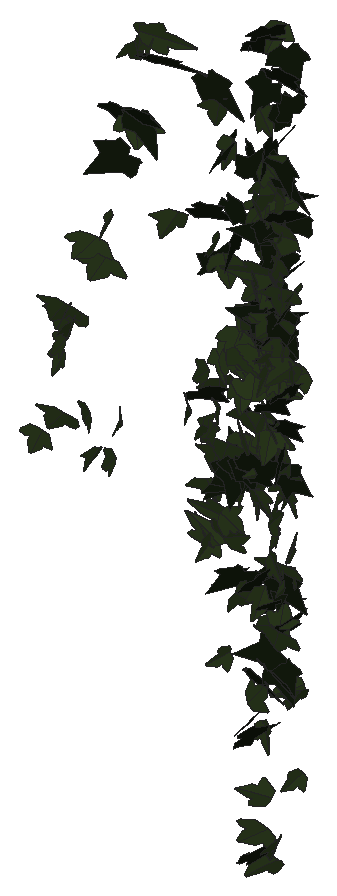
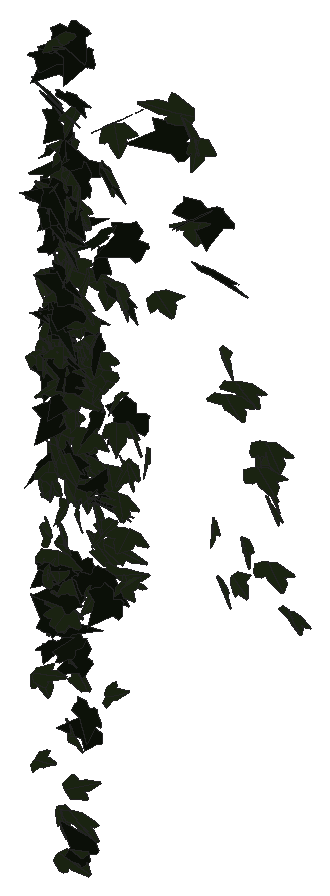
# SketchUp Ruby script. Lengths in millimetres.
U = 1.mm
M = Sketchup.active_model
def pt(a) = Geom::Point3d.new(a.map { |v| v * U })
def face(e, loops, mat)
  f = e.add_face(loops[0].map { |a| pt(a) })
  loops[1..].each { |l| e.add_face(l.map { |a| pt(a) }).erase! }
  f.material = f.back_material = mat if mat
  f
end
# faces: each face lists its corners as indices into pts; further lists are holes
def faces(e, pts, list, mat = nil) = list.each { |f| face(e, (f[0].is_a?(Array) ? f : [f]).map { |l| l.map { |i| pts[i] } }, mat) }
# xy, xz, yz: faces in a plane at the given z, y or x. An outline is a flat list of corners, or four numbers for a rectangle; further outlines are holes
def ring(l) = l.size == 4 ? [[l[0], l[1]], [l[2], l[1]], [l[2], l[3]], [l[0], l[3]]] : l.each_slice(2).to_a
def flat(e, list, mat, &to3) = list.each { |f| face(e, (f[0].is_a?(Array) ? f : [f]).map { |l| ring(l).map { |u, v| to3.(u, v) } }, mat) }
def xy(e, z, list, mat = nil) = flat(e, list, mat) { |x, y| [x, y, z] }
def xz(e, y, list, mat = nil) = flat(e, list, mat) { |x, z| [x, y, z] }
def yz(e, x, list, mat = nil) = flat(e, list, mat) { |y, z| [x, y, z] }
def lines(e, pts, list) = list.each { |a, b| e.add_line(pt(pts[a]), pt(pts[b])) }
# prism: a flat outline (further loops are holes) pulled along v
def prism(e, loops, v, mat = nil)
  f = face(e, loops, mat); d = Geom::Vector3d.new(v.map { |x| x * U })
  f.pushpull(f.normal.samedirection?(d) ? d.length : -d.length)
end
def box(e, o, s, mat = nil) = prism(e, [[o, [o[0] + s[0], o[1], o[2]], [o[0] + s[0], o[1] + s[1], o[2]], [o[0], o[1] + s[1], o[2]]]], [0, 0, s[2]], mat)
def at(x, y, z, deg = 0) = Geom::Transformation.translation(pt([x, y, z])) * Geom::Transformation.rotation(ORIGIN, Z_AXIS, deg.degrees)
def axes(o, x, y, z) = Geom::Transformation.new([*x, 0, *y, 0, *z, 0, *pt(o).to_a, 1])
def part(name) = M.definitions.add(name)
# library, detail: a bought-in or finely detailed component or shape, given as its bounding box
def library(name, o, s) = part(name).tap { |d| box(d.entities, o, s) }
def detail(e, o, s) = box(e.add_group.entities, o, s)
def put(e, d, t, mat = nil) = e.add_instance(d, t).tap { |i| i.material = mat if mat }
def group(e, t, mat = nil) = e.add_group.tap { |g| g.transformation = t; g.material = mat if mat }.entities
root = M.entities
M.materials.add("efeu1").color = [18, 25, 13]
M.materials.add("efeu2").color = [43, 57, 29]
c1 = part("ivyleaf_10")
p = [[0,12.8,-0.8],[-1.5,51.3,-10.9],[-4.9,51,-11.6],[-13.6,26.5,-7.3],[-13.2,15.9,-4.6],[-21.1,19.3,-7.2],
  [-29.5,16.3,-8.3],[-29.2,8.3,-6.2],[-19.7,-9.8,0.5],[-7.6,-13,4],[1,-12.2,5.8],[-0.4,51.1,-11.1],
  [-1.5,51.1,-10.9],[1,-12.4,5.9],[16.9,-12.4,3.5],[35.1,9.1,-5.1],[35,12.9,-6.1],[20.5,16.4,-4.9],
  [15.8,15,-3.8],[15.3,27.6,-7.1],[12.8,31.3,-7.8]]
faces(c1.entities,p,[[0,1,2,3,4,5,6,7,8,9,10],[11,12,0,13,14,15,16,17,18,19,20]],"efeu2")
c2 = part("ivyleaf_9")
p = [[39.1,54.8,31.7],[34.5,51.8,30.2],[-5.3,25.2,17.3],[-17.9,28.3,20.9],[-21.6,21.7,17],[-20.2,4.3,5.3],
  [-22.9,-0.3,2.5],[-17.1,-4,-0.6],[-2,-2.1,-1.2],[-0.7,-15.4,-10.1],[16.6,-22.3,-16.7],[21.1,-15.1,-12.5],
  [32.7,-10.7,-11],[46.1,-1.8,-6.6],[30.8,11.2,3.8]]
faces(c2.entities,p,[[0,1,2,3,4,5,6,7,8,9,10,11,12,13,14]],"efeu1")
put(root,c1,axes([248.1,1016.7,781.5],[1.11617,-0.26381,-0.03342],[-0.05431,0.01802,-0.64306],[0.50317,0.58715,0.00472]))
put(root,c1,axes([302.4,1003.7,838.1],[-1.13074,-0.11611,0.28646],[-0.5208,-0.09105,-0.60444],[0.27356,-0.65326,0.03333]))
put(root,c1,axes([310.2,1017.7,1008.5],[-1.08427,-0.26439,0.28808],[-0.42365,-0.19924,-0.62307],[0.61181,-0.60652,0.0791]))
put(root,c1,axes([319,988.3,1036.9],[-1.20348,-0.11839,0.28705],[-0.52973,-0.07257,-0.64307],[0.26195,-0.69065,0.01836]))
put(root,c1,axes([310.3,993.2,971.9],[0.59347,-0.58954,-0.18764],[-0.17964,0.16234,-0.66689],[1.1637,0.32572,-0.00725]))
put(root,c1,axes([303.6,997.9,945.3],[0.81962,-0.5271,0.10645],[0.12745,-0.08274,-0.68066],[1.01546,0.43583,-0.00049]))
put(root,c1,axes([316.5,987.5,1006.8],[0.23323,-0.35746,0.58793],[-0.42421,0.54436,0.37743],[-1.23892,-0.25368,-0.01856]))
put(root,c1,axes([329.5,990.8,1011.1],[-0.04016,-0.68119,-0.18478],[0.0376,0.18422,-0.68138],[1.34276,-0.02553,0.01355]))
put(root,c1,axes([349.4,1016.5,1147.1],[1.26376,0.10501,-0.25821],[-0.48344,-0.04675,-0.67224],[-0.21846,0.71092,-0.00607]))
put(root,c1,axes([355.1,998.8,860.9],[0.61942,-0.42345,-0.42045],[-0.18112,0.43596,-0.51273],[1.12116,0.30437,0.14946]))
put(root,c1,axes([364.6,1007.5,796.3],[-0.00542,-0.61174,0.26083],[0.04318,-0.26077,-0.61135],[1.26494,0.00628,0.02199]))
put(root,c1,axes([369.2,1018.9,1118.9],[1.27597,0.1776,-0.19159],[-0.38015,0.00838,-0.6912],[-0.32044,0.69722,0.05711]))
put(root,c1,axes([378.8,1020.4,1192.9],[0.41379,-0.70934,0.01301],[0.01004,-0.01199,-0.74191],[1.3502,0.21747,0.00153]))
put(root,c1,axes([388.5,1015.6,787.8],[0.53877,-0.51776,-0.30381],[-0.24959,0.27445,-0.58991],[1.11492,0.31164,0.01475]))
put(root,c2,axes([422.4,1007.7,1322.8],[-1.45679,0.03807,-0.01605],[0.02314,-0.07694,-0.76259],[-0.07514,-0.76173,0.07623]))
put(root,c1,axes([416.7,997.9,872.6],[0.1523,-0.47649,-0.4878],[0.00244,0.49125,-0.47965],[1.2978,0.05499,0.05815]))
put(root,c2,axes([437.6,989.5,1413.5],[1.0707,0.38922,-0.38732],[-0.64433,-0.19072,-0.68339],[-0.82279,0.65585,0.03114]))
put(root,c1,axes([447.6,996.2,1528.7],[-0.32996,-0.70311,-0.34039],[0.25382,0.31691,-0.72254],[1.46489,-0.21328,0.04852]))
put(root,c1,axes([443,1003.2,1390],[1.10989,0.51667,0.01827],[0.02772,0.0111,-0.77912],[-0.98355,0.58335,-0.00135]))
put(root,c2,axes([450.6,1004.7,1400.8],[0.12775,-0.76254,-0.11629],[-0.02111,0.11576,-0.76549],[1.4679,0.06803,-0.00089]))
put(root,c1,axes([472.9,993.3,1553],[0.83085,-0.61324,-0.29097],[-0.24847,0.26363,-0.75151],[1.26772,0.45359,0.0434]))
put(root,c1,axes([508.9,1015.5,1246.3],[-0.61335,-0.59092,0.32145],[-0.0355,-0.34845,-0.65925],[1.27978,-0.29287,0.13577]))
put(root,c2,axes([483.7,990.6,1520],[1.35966,0.01714,0.37317],[0.67839,0.20969,-0.69203],[-0.21273,0.77824,0.17824]))
put(root,c1,axes([489.7,983.5,1563.2],[0.02519,-0.05693,0.81801],[1.34557,0.41521,0.01746],[-0.79053,0.70492,0.05578]))
put(root,c1,axes([551.3,991.7,946.3],[0.37531,-0.48675,-0.48127],[0.05567,0.50638,-0.50016],[1.30156,0.1187,0.16017]))
put(root,c1,axes([562.2,1018.6,998.5],[0.53103,-0.56461,-0.35008],[-0.30438,0.31145,-0.62977],[1.22718,0.32157,-0.00471]))
put(root,c1,axes([573.5,1016.3,714.7],[-0.58884,0.56323,-0.31644],[-0.40676,0.24187,0.63946],[1.16031,0.37062,0.06358]))
put(root,c1,axes([587.8,1009.5,726.6],[0.94751,0.21772,0.48822],[-0.94336,-0.06182,0.53302],[0.38099,-0.69455,0.1056]))
put(root,c1,axes([570,1019,810.8],[-0.98291,-0.35862,-0.18748],[0.33341,0.07588,-0.62772],[0.69426,-0.54416,0.03603]))
put(root,c1,axes([583.2,1019.7,1227.4],[0.29088,-0.72412,-0.07115],[-0.014,0.07116,-0.74003],[1.3847,0.15283,0.00746]))
put(root,c1,axes([589.4,1017.6,865.8],[-1.21967,0.08234,0.16507],[-0.32864,-0.0579,-0.64152],[-0.12347,-0.65923,0.07696]))
put(root,c1,axes([577.8,1001.3,919.1],[-0.19556,-0.42425,-0.55999],[0.33923,0.53169,-0.43552],[1.29334,-0.2036,0.02956]))
put(root,c1,axes([605.8,1008,770.8],[0.08562,-0.04104,-0.7294],[-1.26285,0.30345,-0.058],[0.5817,0.6648,-0.01855]))
put(root,c1,axes([585.2,1009.4,718.1],[0.20264,0.40993,-0.5934],[-0.36544,-0.56207,-0.42274],[-1.32309,0.21803,0.02588]))
put(root,c1,axes([587.7,1001.7,918.6],[0.79668,-0.54431,-0.18352],[-0.12145,0.1816,-0.6842],[1.08646,0.41944,0.05808]))
put(root,c1,axes([589.2,1021.4,990.3],[-0.59703,-0.63775,-0.11816],[0.1123,0.10265,-0.71069],[1.22931,-0.31911,0.00754]))
put(root,c2,axes([606.8,994.5,1211.3],[-0.29868,0.73594,0.3292],[-0.39092,0.22688,-0.7455],[-0.90255,-0.34181,0.21396]))
put(root,c1,axes([599.5,1027.4,521.7],[0.12347,0.12347,-0.66154],[-0.48685,-0.6102,-0.13897],[-1.18466,0.26364,-0.01184]))
put(root,c2,axes([593,971.8,994.3],[0.75861,0.58303,0.19841],[0.1139,0.18945,-0.84932],[-0.74268,0.6246,0.07241]))
put(root,c1,axes([602.7,995.4,962.6],[0.46508,-0.32979,-0.5934],[-0.02565,0.62819,-0.35468],[1.2918,0.13121,0.20659]))
put(root,c2,axes([586.8,975.8,1303.1],[0.92188,0.25005,0.36282],[0.39127,0.18181,-0.79325],[-0.36865,0.81827,0.06538]))
put(root,c1,axes([593.6,1016.4,1037],[-0.03254,-0.6732,0.28474],[0.69627,-0.25446,-0.57963],[1.20434,0.12892,0.3428]))
put(root,c1,axes([621.7,1002,897.1],[-1.21695,-0.18104,0.13771],[-0.25109,-0.03952,-0.66456],[0.35265,-0.65289,0.00204]))
put(root,c1,axes([618.1,988.7,1490.2],[-0.67078,-0.60104,0.10204],[-0.07698,-0.08057,-0.81455],[0.73977,-0.55337,0.00776]))
put(root,c2,axes([596.6,989.5,1521.7],[0.51335,-0.67391,-0.34362],[-0.00076,0.36469,-0.71553],[1.43969,0.24048,0.12215]))
put(root,c2,axes([627.7,1011.7,850.1],[-0.96445,-0.15831,0.02287],[-0.02481,-0.01491,-0.80616],[0.19356,-0.79073,0.01062]))
put(root,c2,axes([617.7,997.9,670.7],[0.45912,0.62563,0.35037],[0.21851,0.30113,-0.73009],[-0.84708,0.41677,0.00157]))
put(root,c2,axes([635.4,1016,846.1],[-0.9666,0.01174,0.15186],[-0.18283,-0.20395,-0.76608],[0.03323,-0.78051,0.20246]))
put(root,c2,axes([630.3,999.1,1419.6],[-0.7137,0.44066,-0.32599],[0.30962,-0.20485,-0.73233],[-0.59273,-0.6376,0.00999]))
put(root,c1,axes([620.9,994.3,1219],[0.8928,0.39439,0.16682],[0.09452,0.20292,-0.81959],[-0.5138,0.72263,0.1391]))
put(root,c1,axes([627.4,998.5,1417.6],[0.8449,-0.41807,0.0234],[0.0279,-0.00739,-0.80893],[0.51008,0.6929,0.0055]))
put(root,c1,axes([624.7,998.6,1055.1],[0.1145,0.7266,0.41294],[0.05784,0.41024,-0.73262],[-1.01797,0.10504,0.00482]))
put(root,c2,axes([640.9,1016.9,863.2],[-0.7071,-0.51491,0.24337],[0.25083,0.13465,0.77452],[-0.64797,0.61402,0.03424]))
put(root,c1,axes([638.1,1009.4,825.8],[0.52366,-0.46226,-0.39053],[-0.17671,0.39168,-0.52903],[1.13807,0.27352,0.09755]))
put(root,c1,axes([627.2,1011.7,1071],[0.94629,0.52834,0.15021],[0.1823,0.11611,-0.72544],[-1.02937,0.50626,0.00961]))
put(root,c2,axes([631.4,1008.3,851.4],[-0.14071,-0.76945,0.20891],[-0.01463,-0.20939,-0.77783],[0.97261,-0.11447,0.01852]))
put(root,c1,axes([621,1000.4,742.7],[-0.9768,0.05015,0.53885],[1.01362,-0.08498,0.51519],[0.18277,0.73929,0.02267]))
put(root,c1,axes([637.8,1004.7,1092.6],[0.94927,0.23006,-0.17094],[-0.20342,-0.03892,-0.81133],[-0.28441,0.7957,0.00974]))
put(root,c2,axes([622.6,1007.1,1311.4],[0.81722,-0.56864,-0.2736],[-0.15198,0.27931,-0.70583],[1.19133,0.4257,0.09764]))
put(root,c1,axes([635,982.1,788.6],[0.04543,0.63832,0.49842],[0.05833,0.49635,-0.63923],[-0.98631,0.05875,-0.01485]))
put(root,c2,axes([634.6,1005.7,993.9],[0.74437,-0.24442,-0.40215],[-0.42811,0.20244,-0.65545],[0.38255,0.70214,0.04899]))
put(root,c2,axes([646.2,1005.2,1120.8],[0.55246,0.09373,-0.6358],[-0.78284,0.02251,-0.4537],[-0.04378,0.78026,0.08946]))
put(root,c2,axes([639,1003.9,1264.4],[-0.26502,0.20492,-0.73112],[0.65798,-0.49364,-0.2986],[-0.65205,-0.58142,-0.00416]))
put(root,c2,axes([656.5,994.3,696.5],[-0.01632,0.34709,-0.68068],[-0.11182,-0.679,-0.3455],[-1.44986,0.04846,0.03431]))
put(root,c1,axes([644,1013.5,1094.8],[0.30714,-0.65765,0.35181],[-0.15798,0.32712,0.70418],[-0.8961,-0.28309,-0.00357]))
put(root,c1,axes([647.7,1023.4,869.5],[-0.26293,-0.7639,-0.02712],[0.01412,0.02491,-0.7937],[0.93244,-0.21578,0.00438]))
put(root,c2,axes([633.8,1015,865.5],[0.55639,-0.66031,-0.13702],[-0.01318,0.15823,-0.79851],[0.82264,0.44914,0.07988]))
put(root,c1,axes([644.7,1011.9,1124.3],[0.15094,0.70154,0.16436],[-0.0377,0.16742,-0.70501],[-1.37081,0.07264,0.03749]))
put(root,c1,axes([646.6,1013.3,1114.3],[-0.60679,0.64842,-0.01098],[0.0086,-0.01001,-0.72257],[-1.23422,-0.31886,0.00036]))
put(root,c1,axes([652.1,1016,954.7],[-1.27683,-0.12742,-0.14668],[0.2762,0.022,-0.68286],[0.24589,-0.68638,0.00534]))
put(root,c1,axes([651.1,1012.8,911.5],[1.29753,-0.20634,0.0203],[0.03887,-0.00261,-0.71229],[0.39268,0.68206,0.00342]))
put(root,c1,axes([670.5,1018,1018.8],[-0.61512,-0.3307,0.57903],[-0.41888,-0.5545,-0.43954],[1.19797,-0.36369,0.14363]))
put(root,c1,axes([655.9,984.5,665.8],[-0.19873,-0.55678,-0.65136],[0.28679,0.60855,-0.57897],[1.0053,-0.28367,0.03641]))
put(root,c2,axes([675.4,1024.9,1078.7],[-0.92839,0.23429,0.0636],[-0.08268,-0.00408,-0.79587],[-0.2844,-0.76362,0.02377]))
put(root,c1,axes([658.1,987.1,1017.6],[0.48459,0.69147,-0.15025],[-0.10005,-0.14076,-0.73686],[-1.34299,0.25999,0.00068]))
put(root,c1,axes([667.6,986.3,920.9],[-0.61818,0.59166,-0.1416],[-0.11145,0.10819,0.77898],[0.73379,0.51488,-0.00098]))
put(root,c2,axes([646.8,1021.3,1406.2],[0.25459,-0.06172,-0.74778],[0.9112,-0.05708,0.21315],[-0.08747,-0.77425,0.04389]))
put(root,c2,axes([674.1,984.1,449.7],[-0.01829,0.73208,0.27968],[-0.0007,0.27972,-0.73221],[-0.95609,-0.01421,-0.00481]))
put(root,c1,axes([657,988.1,1077],[-0.80974,-0.23206,-0.5165],[0.67248,-0.08268,-0.67118],[0.15809,-0.83694,0.20952]))
put(root,c1,axes([675.3,1007.7,1185.8],[0.9461,-0.47244,-0.27677],[-0.3882,0.18713,-0.68578],[0.96708,0.53731,-0.00452]))
put(root,c1,axes([658.8,1029.2,815.8],[0.39988,-0.42483,0.51244],[0.58767,-0.41384,-0.4697],[1.1223,0.36807,0.06336]))
put(root,c1,axes([697.6,993.5,1220.9],[0.18529,0.11008,-0.76258],[-1.44977,-0.10161,-0.11192],[-0.22009,0.76202,0.09524]))
put(root,c1,axes([669.8,996.8,1216.1],[-0.64699,0.65007,-0.14118],[0.07653,-0.13088,-0.83827],[-0.80796,-0.53296,0.03365]))
put(root,c2,axes([665,984,421.5],[0.01144,0.60199,-0.51412],[-0.02109,0.51419,0.60175],[0.96558,0.0041,0.01924]))
put(root,c1,axes([685.5,1009.2,319],[0.18928,0.21267,0.71147],[-0.50555,-0.57834,0.26324],[0.75177,-0.44247,-0.00211]))
put(root,c1,axes([688.5,1020.9,201.5],[-0.52627,-0.41447,0.49617],[-0.41316,-0.44879,-0.49588],[1.15898,-0.34819,0.04853]))
put(root,c2,axes([691.9,1003.8,895.5],[-0.09494,0.18492,0.73524],[-0.53872,0.58974,-0.19507],[-0.75185,-0.44591,0.04692]))
put(root,c1,axes([688.4,998,263.7],[1.10578,-0.18765,-0.37464],[-0.67892,0.11448,-0.61056],[0.41835,0.68178,-0.00059]))
put(root,c2,axes([667,995.8,208.2],[0.507,0.67091,0.04072],[-0.03056,-0.03238,0.78918],[0.81945,-0.41631,0.00423]))
put(root,c2,axes([699.5,994.8,1146.9],[-0.56724,0.1516,0.60854],[-0.71167,0.17358,-0.48894],[-0.28091,-0.7459,0.0099]))
put(root,c1,axes([683.2,1020.5,856.3],[0.16952,-0.69335,0.14255],[0.06345,-0.1394,-0.69889],[1.34569,0.09391,0.01499]))
put(root,c2,axes([681.2,996.5,1613.1],[0.54611,0.67684,0.04547],[0.0273,0.03971,-0.81147],[-0.82716,0.44818,0.00324]))
put(root,c1,axes([677.2,989.1,1135.6],[-0.79653,0.02002,-0.38554],[0.46702,-0.06458,-0.65161],[-0.06103,-0.75547,0.04548]))
put(root,c2,axes([690.9,980.5,702.2],[0.08654,0.88055,0.03894],[0.02393,0.03748,-0.88325],[-1.07506,0.07172,-0.01653]))
put(root,c1,axes([669.6,1025,423.3],[0.73228,-0.31679,0.534],[0.80505,-0.32614,-0.49826],[0.86505,0.57169,0.01166]))
put(root,c1,axes([671.3,1000.9,1151.3],[-1.08076,-0.13918,-0.48937],[0.92793,0.06068,-0.58303],[0.27667,-0.74718,0.04381]))
put(root,c1,axes([681.9,982.1,1019.3],[0.71478,0.59901,-0.28593],[0.25863,0.25217,0.70679],[1.23649,-0.39902,0.01745]))
put(root,c1,axes([681.1,1002.8,1069.5],[0.97533,0.05348,0.06015],[0.07329,0.00311,-0.80124],[-0.06535,0.80171,-0.0009]))
put(root,c1,axes([694.1,979.4,1351.3],[-0.40922,0.39582,0.64097],[-0.50256,0.49108,-0.51882],[-0.7695,-0.53122,-0.00202]))
put(root,c1,axes([692.2,1015.6,893.8],[-0.32312,-0.68666,0.12516],[-0.06249,-0.12081,-0.70733],[1.32692,-0.1729,-0.00283]))
put(root,c1,axes([692.9,989.9,1333.3],[0.84254,-0.20392,-0.30723],[-0.36118,0.08228,-0.72007],[0.26821,0.75137,-0.00453]))
put(root,c2,axes([692.8,1013.2,1536.9],[-0.87784,-0.19735,-0.20147],[0.24402,0.03213,-0.74581],[0.24257,-0.74652,0.02116]))
put(root,c2,axes([671.6,1008.9,1045.1],[0.59521,0.58664,-0.32179],[0.2575,0.24299,0.76297],[0.77463,-0.53153,-0.00636]))
put(root,c1,axes([698.9,1012.9,880.8],[-0.08196,-0.17047,0.69788],[-0.30007,-0.67984,-0.17579],[1.33392,-0.16341,0.00333]))
put(root,c2,axes([699.8,1010.8,1337.5],[-0.04582,0.59258,-0.4817],[-0.14931,-0.48072,-0.58183],[-0.91963,0.04852,0.11847]))
put(root,c2,axes([685.6,983.5,1393.2],[-0.63286,0.05791,0.59778],[0.6991,-0.18876,0.51555],[0.21936,0.76864,0.08157]))
put(root,c1,axes([699.8,1004.3,1038.1],[1.1863,0.08857,-0.34913],[-0.64974,-0.07721,-0.62909],[-0.21856,0.71025,-0.02485]))
put(root,c1,axes([693.3,996.4,673.5],[0.43832,0.69517,-0.33859],[-0.2585,-0.27055,-0.78031],[-0.90724,0.41294,0.05875]))
put(root,c2,axes([707.8,995.5,1293.8],[-0.34803,-0.11319,0.73747],[-0.83722,-0.27006,-0.30691],[0.35724,-0.74318,-0.0008]))
put(root,c2,axes([673.9,991.4,877.5],[0.03981,0.00481,0.85548],[0.99224,-0.26569,-0.02953],[0.3237,0.81383,-0.01469]))
put(root,c2,axes([703,997.1,1641.7],[-0.03417,0.68229,-0.44682],[-0.1364,-0.44607,-0.67415],[-0.98561,0.03808,0.10878]))
put(root,c1,axes([682.2,987.4,493.2],[0.79207,-0.28052,-0.4279],[0.47688,-0.17413,0.70723],[-0.40278,-0.75782,-0.00412]))
put(root,c1,axes([705.3,994.2,963.6],[-0.69693,0.34205,0.47985],[-0.52234,0.21828,-0.6653],[-0.49398,-0.7134,0.02651]))
put(root,c2,axes([690.4,1002.3,1167.2],[0.81408,0.50259,0.04955],[0.05335,0.02431,-0.83535],[-0.61382,0.66867,-0.00688]))
put(root,c2,axes([708.3,1014.2,1133.7],[-0.45757,0.71976,-0.00582],[-0.00099,-0.00699,-0.81161],[-0.87814,-0.37504,0.00395]))
put(root,c1,axes([694.1,1020.2,1091.2],[0.52453,0.68079,-0.01207],[-0.04964,0.01144,-0.80417],[-0.82921,0.42996,0.0405]))
put(root,c2,axes([682.9,981.8,537.8],[0.95239,-0.20446,0.08123],[0.09583,-0.02069,-0.80698],[0.25071,0.78459,-0.00011]))
put(root,c1,axes([695.8,992.4,1495.9],[0.02658,0.75819,0.25552],[-0.05647,0.25638,-0.7568],[-0.97447,0.00582,0.05083]))
put(root,c1,axes([684.1,1017,958.3],[-0.41725,0.14081,0.71519],[0.82278,-0.23862,0.36949],[0.33741,0.75599,-0.01658]))
put(root,c2,axes([712.5,995,1266.7],[-0.35324,0.59237,0.494],[-0.23822,0.45418,-0.65907],[-0.91036,-0.3487,-0.01922]))
put(root,c1,axes([696.1,1001.9,1132.5],[-0.90425,0.1043,-0.17165],[0.20817,-0.01923,-0.74848],[-0.12927,-0.76056,-0.00461]))
put(root,c1,axes([716.4,993.8,1268.6],[-0.36983,0.13366,-0.74242],[-0.81763,0.31957,0.33117],[0.42246,0.7355,-0.00897]))
put(root,c1,axes([699.3,1002.1,1050.5],[0.08174,0.52433,-0.54232],[-0.16076,-0.52795,-0.52671],[-0.90615,0.14096,0.04452]))
put(root,c1,axes([693.8,984.6,847],[-0.72805,0.20671,-0.33164],[0.37613,-0.12294,-0.63141],[-0.29296,-0.67156,0.01351]))
put(root,c2,axes([718.7,1007.7,1216.3],[-0.20591,0.01522,-0.77787],[-0.93267,-0.15106,0.16292],[-0.17627,0.7815,0.04664]))
put(root,c2,axes([721.2,1009.5,1290.1],[-0.52581,0.24942,0.60677],[-0.6364,0.30999,-0.49794],[-0.48537,-0.67664,-0.00445]))
put(root,c1,axes([702.9,1021.2,1633.4],[0.48027,0.57876,-0.39505],[-0.26437,-0.33036,-0.69993],[-0.81299,0.44933,-0.00577]))
put(root,c1,axes([697,1014.7,624.3],[-0.72548,-0.39368,-0.37778],[0.41987,0.16298,-0.71156],[0.51654,-0.6854,0.04779]))
put(root,c1,axes([700.9,991.8,967],[0.10154,0.67691,-0.4173],[-0.12503,-0.40695,-0.68056],[-0.96205,0.12433,0.0444]))
put(root,c1,axes([701.7,1001.9,1223],[-0.74495,0.62615,0.11501],[-0.07769,0.11004,-0.73806],[-1.20914,-0.39285,-0.02343]))
put(root,c1,axes([709.9,1007.3,1044],[0.42215,-0.25237,-0.641],[-0.2906,0.63865,-0.30428],[1.27849,0.2285,0.14249]))
put(root,c2,axes([711.9,999.1,1121.9],[-0.33829,0.78448,-0.14614],[0.07379,-0.1336,-0.83195],[-0.97072,-0.28354,-0.01231]))
put(root,c1,axes([709.5,1000.5,796.9],[-0.06459,0.04542,0.7806],[-0.44287,0.69153,-0.06486],[-0.84491,-0.36595,-0.02568]))
put(root,c1,axes([708.9,1001.9,1223.5],[-0.70061,0.4899,0.28609],[-0.27513,0.17641,-0.75476],[-0.63509,-0.61686,0.01137]))
put(root,c1,axes([706,1012.4,775.4],[0.53234,-0.51091,-0.11973],[-0.08036,0.10116,-0.6717],[0.63513,0.44102,0.01537]))
put(root,c2,axes([711.3,1012.1,1355.6],[-0.00069,0.76781,-0.18396],[0.00772,-0.18395,-0.76779],[-0.96321,-0.00202,-0.00602]))
put(root,c2,axes([698.3,1006.1,1194.1],[-0.07519,0.78621,-0.26039],[-0.02962,0.25928,0.78861],[1.00998,0.06614,0.00375]))
put(root,c1,axes([712.8,1013.3,718],[-1.35482,-0.03864,0.11786],[-0.22385,-0.00767,-0.71291],[0.07494,-0.72151,0.00127]))
put(root,c2,axes([721,995.8,583.8],[-0.5967,-0.15683,0.60953],[-0.70435,-0.19559,-0.51358],[0.30575,-0.75663,0.00642]))
put(root,c1,axes([713.6,1004.8,1340.8],[0.88715,-0.40228,-0.47354],[-0.22656,0.5232,-0.56164],[1.16064,0.40962,0.25232]))
put(root,c1,axes([705,1007,1181.4],[0.4437,0.69944,-0.01687],[-0.00959,-0.01492,-0.78834],[-0.85351,0.36377,0.00009]))
put(root,c1,axes([711.6,1002.2,1086.5],[-0.43428,-0.67276,-0.14966],[0.1019,0.13987,-0.71039],[1.30774,-0.23431,0.00565]))
put(root,c1,axes([715.4,994.5,1268],[0.5997,-0.52468,-0.39049],[-0.32386,0.28639,-0.71897],[0.72925,0.55866,0.00183]))
put(root,c2,axes([696.1,995.2,648.8],[0.65541,0.08088,0.62448],[0.56244,0.50863,-0.46248],[-0.5233,0.64798,0.28507]))
put(root,c1,axes([708.8,989.9,1381.7],[-0.73743,-0.48908,-0.20865],[0.20818,0.12078,-0.77743],[0.6144,-0.62794,0.01298]))
put(root,c2,axes([705.8,992.2,1003.7],[0.59176,0.57657,0.15317],[0.11644,0.11987,-0.75345],[-0.71844,0.49433,0.00405]))
put(root,c1,axes([709.7,1007.3,939.4],[-0.97199,-0.01289,-0.10164],[0.12477,-0.05234,-0.79502],[0.00749,-0.80147,0.05356]))
put(root,c2,axes([708.1,1020.9,704.6],[-0.66066,-0.45185,-0.36971],[0.33931,0.24371,-0.70523],[0.62625,-0.60872,-0.00792]))
put(root,c1,axes([725,993.4,1149],[-0.97629,-0.34234,0.40403],[-0.46474,-0.34622,-0.60339],[0.89432,-0.55363,0.12751]))
put(root,c1,axes([708.5,1008.1,1116.3],[-0.12449,0.73817,-0.0861],[0.0017,-0.08672,-0.74512],[-0.90668,-0.10152,0.01042]))
put(root,c2,axes([697.4,1002.1,1136.7],[0.3178,0.06632,0.71485],[0.7958,0.29578,-0.26514],[-0.36585,0.70099,0.04424]))
put(root,c2,axes([690.2,1001.2,558.2],[0.63031,-0.63402,0.25519],[0.28075,-0.21058,-0.71462],[1.27008,0.3612,0.03132]))
put(root,c1,axes([716.8,988.8,1256.1],[-1.01434,0.16967,0.09937],[-0.13735,-0.05682,-0.845],[-0.19667,-0.83541,0.07765]))
put(root,c1,axes([708.9,979.9,1369.6],[-0.13016,-0.23752,-0.78971],[0.40634,0.71605,-0.26036],[0.92038,-0.34972,0.00326]))
put(root,c1,axes([724.1,1021,1067.2],[-0.72541,-0.16977,0.33654],[-0.37415,-0.14756,-0.61628],[0.26737,-0.66711,0.05067]))
put(root,c1,axes([713.2,986.8,951.1],[0.64916,0.58455,-0.15723],[-0.12955,-0.11596,-0.79046],[-0.72705,0.54259,0.00046]))
put(root,c1,axes([717.4,1015.5,905.1],[0.79687,-0.37356,-0.23313],[-0.17819,0.20965,-0.74515],[0.5068,0.66109,0.10458]))
put(root,c1,axes([712.6,999.4,1334.1],[0.1577,0.79092,-0.04758],[-0.01392,-0.04634,-0.8014],[-0.96657,0.12971,0.00378]))
put(root,c1,axes([703.5,1010.6,1025.2],[-0.18865,-0.44323,-0.59194],[0.83212,0.44654,-0.40757],[1.13506,-0.40103,0.20041]))
put(root,c2,axes([709.9,996.8,1446],[-0.07527,0.06059,-0.81283],[0.72924,-0.55082,-0.08643],[-0.67605,-0.60091,-0.00273]))
put(root,c1,axes([719.8,992.7,257.2],[-0.02835,-0.72101,-0.11407],[0.01825,0.11389,-0.72113],[1.38918,-0.01621,0.00714]))
put(root,c2,axes([723.8,1021.9,1327.4],[-0.44965,0.59985,-0.325],[0.21919,-0.27102,-0.70396],[-0.80295,-0.4099,-0.01017]))
put(root,c2,axes([731.6,1016.5,1092.2],[-0.88906,0.30952,0.03809],[-0.10224,-0.1011,-0.78171],[-0.36647,-0.72269,0.12567]))
put(root,c1,axes([728.7,991,616.3],[-1.34923,-0.00909,0.18833],[-0.35756,-0.02782,-0.70856],[0.03031,-0.73299,0.02456]))
put(root,c2,axes([737,1001.2,1506.5],[-0.6227,0.43494,0.41114],[-0.43132,0.21689,-0.66835],[-0.58916,-0.61848,0.05475]))
put(root,c2,axes([712.2,1003.9,965.3],[0.82784,0.45146,0.06735],[0.04968,0.06031,-0.81456],[-0.55466,0.67922,0.02756]))
put(root,c1,axes([721.3,1029.6,852.9],[-0.03244,-0.53595,0.46997],[0.06055,-0.47021,-0.53507],[1.35529,0.00818,0.03515]))
put(root,c1,axes([716.6,1004.3,1100.4],[0.80691,-0.50269,0.10098],[0.0994,-0.05968,-0.83075],[0.61759,0.6664,0.00177]))
put(root,c1,axes([716.1,1009.7,626.2],[0.69363,0.31019,-0.12846],[0.13626,0.0635,0.64766],[0.38627,-0.57941,0.00221]))
put(root,c2,axes([710.2,1017.3,606.1],[0.38051,0.68993,0.05468],[-0.05675,-0.03895,0.75669],[0.84244,-0.31425,0.02628]))
put(root,c1,axes([717.6,1027.4,834.9],[0.0161,-0.48023,-0.4668],[0.00353,-0.46685,0.48036],[-0.81705,-0.01148,-0.00712]))
put(root,c2,axes([703.3,1012,1350.7],[0.46104,0.04918,0.66035],[0.79327,0.11624,-0.38076],[-0.15279,0.7519,0.01567]))
put(root,c1,axes([735.3,985,1371.4],[0.06088,-0.09413,-0.86374],[-0.65716,0.67548,-0.10473],[0.83171,0.54061,-0.01953]))
put(root,c1,axes([708.5,1004.5,1212.6],[0.26109,-0.2507,-0.71753],[0.54463,-0.56185,0.32945],[-0.75049,-0.49495,-0.01054]))
put(root,c1,axes([719.8,1027.9,690.1],[-0.00114,-0.16747,0.7103],[0.2352,-0.68513,-0.16128],[0.8587,0.18744,0.04512]))
put(root,c2,axes([736.4,1011.5,1135.6],[-0.87977,0.37351,-0.01669],[-0.06084,-0.13203,-0.79993],[-0.45206,-0.70913,0.14014]))
put(root,c1,axes([748.3,983,1307.8],[0.39001,-0.06423,-0.77113],[-1.34586,0.30834,-0.2136],[0.59793,0.73591,0.02219]))
put(root,c1,axes([731.5,1029.1,512.4],[-0.27743,-0.03849,0.70203],[-0.32513,-0.67806,-0.1235],[0.79376,-0.29119,0.19478]))
put(root,c1,axes([707.2,997.8,734.6],[0.33074,-0.16793,0.71501],[0.82101,-0.24852,-0.31352],[0.35895,0.72317,0.05829]))
put(root,c1,axes([720.5,973,1423.1],[0.14499,0.75242,0.4757],[0.02795,0.47718,-0.76048],[-1.08566,0.11277,0.04395]))
put(root,c1,axes([730.4,996.4,1200.2],[-0.94653,-0.31539,0.09171],[-0.0915,-0.05893,-0.83709],[0.39012,-0.77902,0.02619]))
put(root,c1,axes([728.8,999.3,1112.4],[-0.54847,-0.657,0.04508],[0.05302,-0.08407,-0.79173],[0.80168,-0.44393,0.08321]))
put(root,c1,axes([729,1013.2,868.2],[-0.50696,-0.64167,-0.0647],[0.05613,0.04728,-0.76437],[0.78481,-0.41788,0.01287]))
put(root,c2,axes([717,984.6,1320.7],[-0.12104,-0.26302,-0.75239],[0.22912,0.72913,-0.27966],[0.945,-0.21047,-0.02857]))
put(root,c2,axes([726.6,994.4,1253.1],[-0.50899,-0.32068,0.67833],[0.65642,0.41307,0.52621],[-0.63798,0.68085,0.00024]))
put(root,c2,axes([715.4,1010.7,694.1],[-0.22045,-0.20058,-0.71209],[0.54559,0.55432,-0.26962],[0.71898,-0.48214,-0.01373]))
put(root,c1,axes([722.7,1020,843.3],[-0.54205,0.35213,-0.33427],[0.28396,-0.24318,-0.56553],[-0.51984,-0.50001,0.03963]))
put(root,c2,axes([731.4,984.9,1461.4],[0.21736,0.49731,0.59196],[0.08993,0.59378,-0.52102],[-0.93892,0.17199,0.08713]))
put(root,c2,axes([726.1,1001.7,931.6],[-0.47799,0.17914,-0.64883],[0.72745,-0.25596,-0.43073],[-0.38101,-0.71342,-0.00838]))
put(root,c2,axes([721.7,1019.3,1601.5],[-0.34985,-0.5517,-0.47132],[0.36856,0.37,-0.61691],[0.80487,-0.40923,0.07762]))
put(root,c2,axes([735.8,978.2,1161.1],[0.14726,0.46617,0.65874],[0.02394,0.66418,-0.47361],[-0.98425,0.0859,0.08704]))
put(root,c1,axes([736.6,1024.1,505.6],[-0.4188,-0.58774,0.10559],[-0.07692,-0.09762,-0.62757],[1.13389,-0.2237,-0.00357]))
put(root,c2,axes([734.9,993.4,1033],[0.25386,0.72287,0.17476],[0.05902,0.16793,-0.75222],[-0.90538,0.21363,-0.00003]))
put(root,c1,axes([736.4,1028.2,360.7],[0.21472,0.29213,-0.54169],[-0.34733,-0.46085,-0.34103],[-0.66567,0.33469,0.00321]))
put(root,c1,axes([743.7,997.6,1076.5],[-0.45367,-0.40672,0.63951],[-0.37961,-0.56761,-0.54192],[0.84311,-0.47442,0.10011]))
put(root,c1,axes([722.7,1027.3,697.9],[0.03084,-0.04858,-0.68437],[0.41943,-0.59175,0.05471],[-0.72436,-0.34472,0.00254]))
put(root,c2,axes([725.3,998.4,557],[-0.06288,-0.68036,-0.38634],[0.09017,0.38122,-0.68119],[0.95026,-0.08119,0.03908]))
put(root,c1,axes([731.7,1000.9,1307.7],[0.32714,-0.74457,0.00739],[0.2458,0.02234,-0.75287],[1.39566,0.17059,0.13086]))
put(root,c2,axes([745.8,1006.1,1335],[-1.40251,-0.22496,-0.02987],[0.05454,0.00844,-0.77049],[0.42845,-0.73748,0.00029]))
put(root,c1,axes([735.6,1007,745.6],[0.37087,-0.53536,0.41652],[-0.25142,0.36196,0.61565],[-0.78841,-0.36726,-0.0004]))
put(root,c2,axes([726.2,998.6,1155.1],[0.20733,-0.72031,-0.40589],[-0.11942,0.39394,-0.74007],[1.0016,0.19607,-0.00421]))
put(root,c1,axes([739.3,996.4,1079.6],[0.82653,-0.41529,-0.4035],[-0.21809,0.43276,-0.56874],[1.08022,0.40513,0.19391]))
put(root,c1,axes([718.6,994.8,1341.1],[0.54539,0.04825,-0.66928],[0.78533,0.19622,0.44411],[0.23113,-0.78056,0.07027]))
put(root,c1,axes([724.7,1029.7,1053.8],[-0.29292,0.20508,0.71295],[0.64961,-0.47415,0.31571],[0.63021,0.58406,0.00595]))
put(root,c2,axes([751.4,994.2,1519.1],[-0.16656,0.53416,0.54564],[-0.51077,0.41118,-0.50728],[-0.77905,-0.38379,0.21593]))
put(root,c2,axes([730.8,1009,883.3],[0.35342,-0.30983,-0.64966],[-0.33514,0.5997,-0.4085],[0.81164,0.38254,0.11422]))
put(root,c2,axes([724.7,985.5,1580.6],[0.97408,0.15118,0.0487],[0.05854,0.00835,-0.81262],[-0.18472,0.79987,-0.00073]))
put(root,c2,axes([717.6,1001.7,1400.8],[0.66317,-0.69807,-0.06702],[0.02797,0.08209,-0.77862],[1.33438,0.34521,0.04963]))
put(root,c1,axes([748.5,1018.2,1058.3],[0.58464,-0.00739,-0.60101],[-0.73238,0.03252,-0.47905],[0.03664,0.76799,0.0145]))
put(root,c1,axes([740.4,1017.4,1197.5],[0.24129,-0.72667,0.12442],[-0.00161,-0.12639,-0.73731],[1.40311,0.12482,-0.02224]))
put(root,c2,axes([724.6,997.3,1427.4],[0.10561,-0.75516,0.22128],[0.02341,-0.22097,-0.75719],[1.49748,0.05671,-0.00377]))
put(root,c2,axes([739,983,1343.3],[0.51716,0.64776,-0.12364],[-0.09474,-0.09693,-0.77404],[-0.79893,0.43079,0.01175]))
